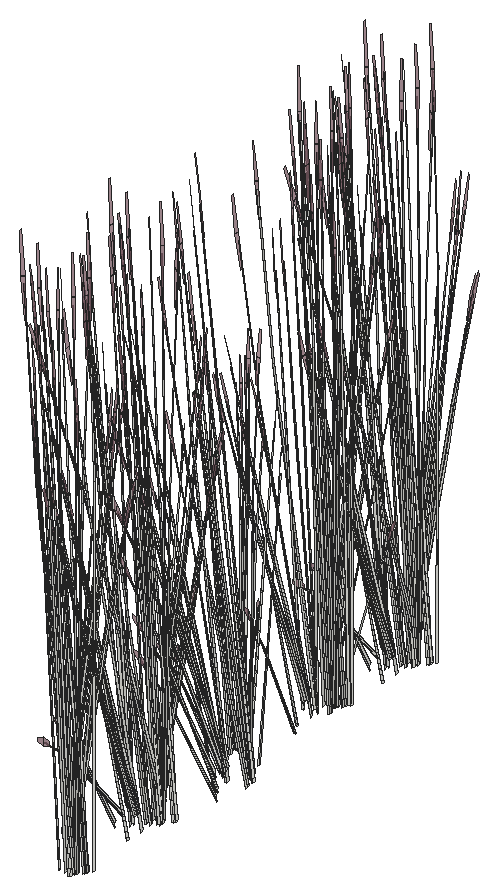
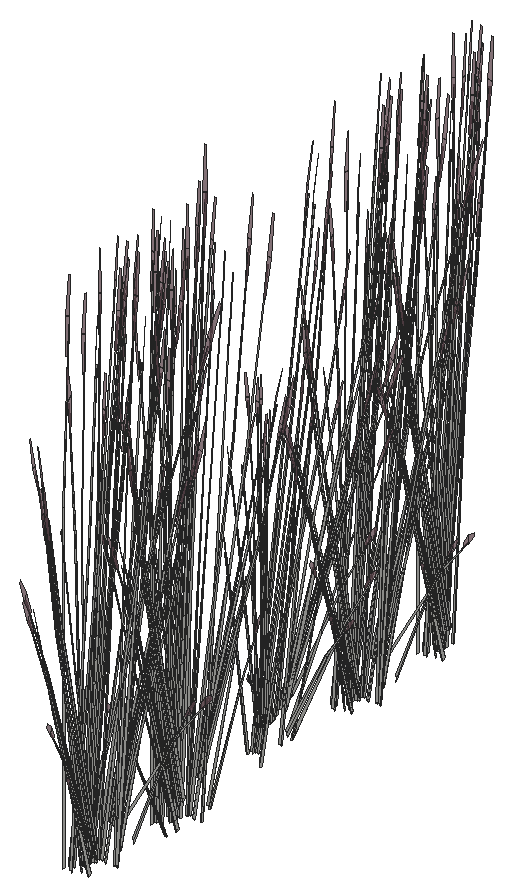
# SketchUp Ruby script. Lengths in inches.
U = 1.inch
M = Sketchup.active_model
def pt(a) = Geom::Point3d.new(a.map { |v| v * U })
def face(e, loops, mat)
  f = e.add_face(loops[0].map { |a| pt(a) })
  loops[1..].each { |l| e.add_face(l.map { |a| pt(a) }).erase! }
  f.material = f.back_material = mat if mat
  f
end
# faces: each face lists its corners as indices into pts; further lists are holes
def faces(e, pts, list, mat = nil) = list.each { |f| face(e, (f[0].is_a?(Array) ? f : [f]).map { |l| l.map { |i| pts[i] } }, mat) }
# xy, xz, yz: faces in a plane at the given z, y or x. An outline is a flat list of corners, or four numbers for a rectangle; further outlines are holes
def ring(l) = l.size == 4 ? [[l[0], l[1]], [l[2], l[1]], [l[2], l[3]], [l[0], l[3]]] : l.each_slice(2).to_a
def flat(e, list, mat, &to3) = list.each { |f| face(e, (f[0].is_a?(Array) ? f : [f]).map { |l| ring(l).map { |u, v| to3.(u, v) } }, mat) }
def xy(e, z, list, mat = nil) = flat(e, list, mat) { |x, y| [x, y, z] }
def xz(e, y, list, mat = nil) = flat(e, list, mat) { |x, z| [x, y, z] }
def yz(e, x, list, mat = nil) = flat(e, list, mat) { |y, z| [x, y, z] }
def lines(e, pts, list) = list.each { |a, b| e.add_line(pt(pts[a]), pt(pts[b])) }
# prism: a flat outline (further loops are holes) pulled along v
def prism(e, loops, v, mat = nil)
  f = face(e, loops, mat); d = Geom::Vector3d.new(v.map { |x| x * U })
  f.pushpull(f.normal.samedirection?(d) ? d.length : -d.length)
end
def box(e, o, s, mat = nil) = prism(e, [[o, [o[0] + s[0], o[1], o[2]], [o[0] + s[0], o[1] + s[1], o[2]], [o[0], o[1] + s[1], o[2]]]], [0, 0, s[2]], mat)
def at(x, y, z, deg = 0) = Geom::Transformation.translation(pt([x, y, z])) * Geom::Transformation.rotation(ORIGIN, Z_AXIS, deg.degrees)
def axes(o, x, y, z) = Geom::Transformation.new([*x, 0, *y, 0, *z, 0, *pt(o).to_a, 1])
def part(name) = M.definitions.add(name)
# library, detail: a bought-in or finely detailed component or shape, given as its bounding box
def library(name, o, s) = part(name).tap { |d| box(d.entities, o, s) }
def detail(e, o, s) = box(e.add_group.entities, o, s)
def put(e, d, t, mat = nil) = e.add_instance(d, t).tap { |i| i.material = mat if mat }
def group(e, t, mat = nil) = e.add_group.tap { |g| g.transformation = t; g.material = mat if mat }.entities
root = M.entities
M.materials.add("LightPink_Translucent").color = [144, 107, 117]
M.materials["LightPink_Translucent"].alpha = 0.75
c1 = part("blade")
p = [[2.15,0.21,22],[0,0.17,0],[0.09,0.45,0],[2.18,0.31,22],[2.29,0.31,22],[0.38,0.45,0],
  [2.48,0.24,33],[2.49,0.24,33],[2.48,0.22,33]]
faces(c1.entities,p,[[0,1,2,3],[4,5,2,3],[6,3,4,7],[8,0,3,6]])
c2 = part("seeds")
p = [[0.3,-0.1,1.38],[-0.01,-0.03,1.59],[-0.01,-0.03,0.03],[0.14,-0.07,-0.07],[0.29,-0.03,3],[0.15,0.01,3.11]]
faces(c2.entities,p,[[0,1,2,3],[1,0,4,5]],"LightPink_Translucent")
c3 = part("blade with seeds")
put(c3.entities,c1,at(0,0,0))
put(c3.entities,c2,axes([2.4,0.25,30.99],[1.5799,-0.05474,1.17369],[-0.12525,1.92788,0.29478],[-0.07173,-0.02425,1.56792]))
put(root,c3,axes([402.67,375.75,-9.47],[-0.24813,0.48978,0.41661],[-0.51557,-0.23571,-0.2005],[0,-0.1129,1.33761]))
put(root,c3,axes([402.84,375.87,-9.8],[0.64638,0.11452,0.42607],[-0.13155,0.64678,0.16719],[-0.09446,-0.06245,1.47927]))
put(root,c3,axes([402.49,376.9,-9.7],[0.54955,-0.14427,0.16428],[0.1357,0.53689,0.32672],[-0.04901,-0.07823,1.49371]))
put(root,c3,axes([403,376.33,-9.5625],[-0.09866,0.48509,0.13483],[-0.48202,-0.0842,-0.38503],[-0.08772,-0.04981,1.18024]))
put(root,c3,axes([404.125,376.93,-9.7],[0.14774,-0.54019,0.16428],[0.54062,0.15287,0.32672],[-0.09339,0.00263,1.49371]))
put(root,c3,axes([403.2,376.99,-9.95],[-0.51557,-0.24403,0],[0.24813,-0.50705,0],[0,0,1.51513]))
put(root,c3,axes([403.625,376.34,-9.7],[-0.49938,-0.43748,-0.23459],[0.42021,-0.49126,0.51337],[-0.13447,0.05118,1.56642]))
put(root,c3,axes([402.31,377.18,-9.69],[0.47863,0.27177,0.46235],[-0.28609,0.48733,0],[-0.10901,-0.0619,1.46668]))
put(root,c3,axes([403.37,376.24,-9.94],[-0.55535,0.03355,-0.41661],[-0.05022,-0.55698,0.2005],[-0.09942,0.05645,1.33761]))
put(root,c3,axes([403.99,377.54,-9.96],[-0.31576,-0.54657,-0.04789],[0.53494,-0.30375,0.48057],[-0.13182,0.05204,1.52373]))
put(root,c3,axes([403.875,376.21,-9.5625],[0.37783,0.32657,0.13483],[-0.31516,0.36844,-0.38503],[-0.08772,0.04981,1.18024]))
put(root,c3,axes([403.84,377.47,-10.11],[-0.47712,-0.13449,-0.28847],[0.12013,-0.47362,0.28847],[-0.09619,0.05462,1.29413]))
put(root,c3,axes([403.76,376.09,-9.52],[0.05959,0.62022,-0.27094],[-0.62068,0.0375,-0.46562],[-0.1093,0.08261,1.4872]))
put(root,c3,axes([403.95,377.68,-10.12],[-0.47863,0.27177,-0.46235],[-0.28609,-0.48733,0],[-0.10901,0.0619,1.46668]))
put(root,c3,axes([403.22,382.96,-7.61],[-0.07822,-0.07621,1.62908],[-0.52201,0.04832,-0.25764],[-0.08331,-0.18228,0.13065]))
put(root,c3,axes([401.8,377.02,-7.3],[0.34603,-0.28618,0.32977],[0.32756,0.32677,-0.42575],[-0.04984,0.16603,0.81462]))
put(root,c3,axes([403.77,384.25,-7.36],[-0.24409,-0.44196,-0.66157],[0.50245,-0.2463,0.07984],[-0.05708,-0.21354,0.93586]))
put(root,c3,axes([404.39,377.6,-9.79],[0.31974,0.54466,0],[-0.53494,0.30375,-0.48057],[-0.12184,0.06918,1.52448]))
put(root,c3,axes([404.12,375.44,-9.35],[-0.01397,-0.51177,1.31553],[0.63227,0.13266,0.557],[-0.14954,0.28003,1.24175]))
put(root,c3,axes([403.58,384.16,-7.64],[-0.50273,-0.13626,-0.47583],[0.17232,-0.46717,-0.36857],[-0.0461,-0.18809,0.91046]))
put(root,c3,axes([402.63,377.87,-7.6],[-0.37684,0.18473,0.05988],[-0.18445,-0.33686,0.47138],[0.03639,0.14849,0.71878]))
put(root,c3,axes([401.58,377.1,-6.97],[0.56206,0.02693,-0.12569],[-0.01536,0.50991,-0.69765],[-0.03904,0.19638,1.06006]))
put(root,c3,axes([402.58,383.87,-7.26],[0.56969,-0.13971,0.50064],[0.09887,0.54803,0.4128],[-0.13398,-0.16152,1.03595]))
put(root,c3,axes([402.76,377.83,-7.28],[-0.50393,-0.1421,0.49617],[0.17232,-0.46717,0.40911],[0.03028,0.18372,1.0267]))
put(root,c3,axes([401.84,378.54,-9.42],[-0.01324,-0.32319,1.06958],[0.33072,0.23052,0.78586],[-0.06504,0.15405,0.23558]))
put(root,c3,axes([404.01,384.14,-7.3125],[-0.50045,0.25306,-0.11324],[-0.24593,-0.44915,-0.62851],[-0.06603,-0.18927,0.95501]))
put(root,c3,axes([402.02,383.37,-9.42],[0.26677,0.18918,1.06958],[-0.38851,0.11372,0.78586],[-0.08313,-0.14539,0.23558]))
put(root,c3,axes([401.96,377.29,-7.34],[0.3661,0.36521,-0.52818],[-0.38674,0.31985,-0.40911],[-0.0557,0.18556,1.01061]))
put(root,c3,axes([401.5625,377.84,-9.37],[0.46459,-0.09625,0.0606],[0.10681,0.38778,-0.80367],[-0.02945,0.1963,0.72038]))
put(root,c3,axes([402.71,383.99,-7.6],[0.23243,-0.34529,0.05988],[0.331,0.20103,0.47138],[-0.10701,-0.1107,0.71878]))
put(root,c3,axes([402.64,385.91,-10.05],[-0.21003,-0.55738,-0.65031],[0.60499,-0.20074,-0.17068],[-0.02321,-0.18874,1.43544]))
put(root,c3,axes([401.85,377.12,-7.03],[-0.01331,0.50278,-0.73435],[-0.56035,-0.03377,0.08862],[-0.05914,0.213,1.03881]))
put(root,c3,axes([402.38,376.76,-8.39],[-0.01252,-0.20862,1.59586],[0.54251,0.1384,0.12904],[-0.03356,0.2973,0.68222]))
put(root,c3,axes([403.26,383.65,-10.02],[-0.35341,0.31182,-0.03625],[-0.32382,-0.34152,-0.16435],[-0.0228,-0.09677,0.54209]))
put(root,c3,axes([403.71,387.35,-8.9],[0.44194,0.21918,1.40854],[-0.43295,0.47219,0.557],[-0.19393,-0.27986,1.18082]))
put(root,c3,axes([402.78,384.39,-7.3],[0.07899,0.43781,0.32977],[-0.45153,0.11561,-0.42575],[-0.12128,-0.12546,0.81462]))
put(root,c3,axes([401.4,385.83,-10.12],[0,-0.54355,-0.46235],[0.57217,0,0],[0,-0.1238,1.46668]))
put(root,c3,axes([401.66,377.83,-8.87],[0.01124,-0.2806,1.43727],[0.50537,0.14821,0.19862],[-0.04379,0.29905,0.67868]))
put(root,c3,axes([401.65,385.84,-10.11],[0.35699,-0.33913,-0.28847],[0.35699,0.33913,0.28847],[0,-0.10923,1.29413]))
put(root,c3,axes([402.9,386.46,-9.52],[-0.57594,-0.25935,-0.27094],[0.27732,-0.5474,-0.46562],[-0.0181,-0.1344,1.4872]))
put(root,c3,axes([401.75,386.08,-9.83],[-0.47569,0.45698,0.2864],[-0.47598,-0.45217,-0.33981],[-0.01661,-0.12977,1.53541]))
put(root,c3,axes([403.04,387.04,-9.73],[0.13555,-0.64407,-0.21817],[0.64269,0.11227,0.47743],[-0.1123,-0.08895,1.45677]))
put(root,c3,axes([401.65,386.34,-9.69],[0,0.54355,0.46235],[-0.57217,0,0],[0,-0.1238,1.46668]))
put(root,c3,axes([403,386.78,-9.94],[-0.30722,-0.45622,-0.41661],[0.46535,-0.32126,0.2005],[-0.09942,-0.05645,1.33761]))
put(root,c3,axes([402.95,386.61,-9.47],[-0.24813,0.48978,0.41661],[-0.51557,-0.23571,-0.2005],[0,-0.1129,1.33761]))
put(root,c3,axes([403.12,386.73,-9.8],[0.64638,0.11452,0.42607],[-0.13155,0.64678,0.16719],[-0.09446,-0.06245,1.47927]))
put(root,c3,axes([402.77,387.76,-9.7],[0.54955,-0.14427,0.16428],[0.1357,0.53689,0.32672],[-0.04901,-0.07823,1.49371]))
put(root,c3,axes([403.28,387.1875,-9.5625],[-0.09866,0.48509,0.13483],[-0.48202,-0.0842,-0.38503],[-0.08772,-0.04981,1.18024]))
put(root,c3,axes([403.9,387.2,-9.7],[-0.49938,-0.43748,-0.23459],[0.42021,-0.49126,0.51337],[-0.13447,0.05118,1.56642]))
put(root,c3,axes([402.59,388.03,-9.69],[0.47863,0.27177,0.46235],[-0.28609,0.48733,0],[-0.10901,-0.0619,1.46668]))
put(root,c3,axes([403.65,387.1,-9.94],[-0.55535,0.03355,-0.41661],[-0.05022,-0.55698,0.2005],[-0.09942,0.05645,1.33761]))
put(root,c3,axes([404.27,388.4,-9.96],[-0.31576,-0.54657,-0.04789],[0.53494,-0.30375,0.48057],[-0.13182,0.05204,1.52373]))
put(root,c3,axes([404.12,388.33,-10.11],[-0.47712,-0.13449,-0.28847],[0.12013,-0.47362,0.28847],[-0.09619,0.05462,1.29413]))
put(root,c3,axes([404.63,393.81,-8.39],[0.1169,0.17452,1.59586],[-0.54019,0.14692,0.12904],[-0.12209,-0.27397,0.68222]))
put(root,c3,axes([404.04,386.95,-9.52],[0.05959,0.62022,-0.27094],[-0.62068,0.0375,-0.46562],[-0.1093,0.08261,1.4872]))
put(root,c3,axes([404.49,393.34,-9.59],[-0.03097,0.17781,1.33163],[-0.45273,0.14885,-0.28638],[-0.10583,-0.22982,0.56934]))
put(root,c3,axes([403.67,387.43,-10.08],[-0.34446,0.40855,-0.58063],[-0.42791,-0.37046,-0.15239],[-0.13803,0.10191,1.28164]))
put(root,c3,axes([404.24,388.54,-10.12],[-0.47863,0.27177,-0.46235],[-0.28609,-0.48733,0],[-0.10901,0.0619,1.46668]))
put(root,c3,axes([404.99,392.4,-7.62],[-0.00954,0.06515,1.65179],[-0.47055,0.23645,-0.15608],[-0.13847,-0.12087,0.29231]))
put(root,c3,axes([402.08,387.88,-7.3],[0.34603,-0.28618,0.32977],[0.32756,0.32677,-0.42575],[-0.04984,0.16603,0.81462]))
put(root,c3,axes([404.4,386.3,-9.35],[-0.01397,-0.51177,1.31553],[0.63227,0.13266,0.557],[-0.14954,0.28003,1.24175]))
put(root,c3,axes([404.97,394.0625,-7.36],[-0.43608,-0.26272,-0.66157],[0.30991,-0.46038,0.07984],[-0.158,-0.15687,0.93586]))
put(root,c3,axes([404.82,393.71,-7.78],[-0.07899,-0.43781,-0.32977],[0.45153,-0.11561,0.42575],[-0.12128,-0.12546,0.81462]))
put(root,c3,axes([404.12,393.63,-10.61],[-0.04954,0.0716,1.6421],[-0.50062,0.15438,-0.25086],[-0.12094,-0.14044,0.2797]))
put(root,c3,axes([404.77,394.07,-7.64],[-0.50465,0.12921,-0.47583],[-0.08828,-0.48932,-0.36857],[-0.13555,-0.14022,0.91046]))
put(root,c3,axes([401.86,387.96,-6.97],[0.56206,0.02693,-0.12569],[-0.01536,0.50991,-0.69765],[-0.03904,0.19638,1.06006]))
put(root,c3,axes([405.12,393.64,-6.94],[-0.34131,0.52108,-0.12682],[-0.49429,-0.3002,-0.70393],[-0.17182,-0.14722,1.06961]))
put(root,c3,axes([402.12,389.39,-9.42],[-0.01324,-0.32319,1.06958],[0.33072,0.23052,0.78586],[-0.06504,0.15405,0.23558]))
put(root,c3,axes([402.24,388.15,-7.34],[0.3661,0.36521,-0.52818],[-0.38674,0.31985,-0.40911],[-0.0557,0.18556,1.01061]))
put(root,c3,axes([401.84,388.7,-9.37],[0.46459,-0.09625,0.0606],[0.10681,0.38778,-0.80367],[-0.02945,0.1963,0.72038]))
put(root,c3,axes([403.73,394.36,-7.26],[0.42234,-0.40113,0.50064],[0.36424,0.42599,0.4128],[-0.19815,-0.07399,1.03595]))
put(root,c3,axes([402.13,387.98,-7.03],[-0.01331,0.50278,-0.73435],[-0.56035,-0.03377,0.08862],[-0.05914,0.213,1.03881]))
put(root,c3,axes([400.66,389.3,-7.62],[0.05802,-0.03282,1.65179],[0.47954,0.21828,-0.15608],[-0.01127,0.18175,0.29231]))
put(root,c3,axes([402.66,387.625,-8.39],[-0.01252,-0.20862,1.59586],[0.54251,0.1384,0.12904],[-0.03356,0.2973,0.68222]))
put(root,c3,axes([403.93,394.35,-7.6],[0.02575,-0.41332,0.05988],[0.38885,0.01133,0.47138],[-0.14895,-0.04325,0.71878]))
put(root,c3,axes([403.81,393.9,-10.02],[-0.14753,0.44383,-0.03625],[-0.45406,-0.13653,-0.16435],[-0.06894,-0.07259,0.54209]))
put(root,c3,axes([403.5625,395.93,-9.79],[-0.63949,0,0],[0,-0.60749,-0.48057],[0,-0.13836,1.52448]))
put(root,c3,axes([401.94,388.6875,-8.87],[0.01124,-0.2806,1.43727],[0.50537,0.14821,0.19862],[-0.04379,0.29905,0.67868]))
put(root,c3,axes([404.19,394.66,-7.3],[0.29098,0.34031,0.32977],[-0.33226,0.32215,-0.42575],[-0.16881,-0.04902,0.81462]))
put(root,c3,axes([403.08,395.3,-9.42],[0.3265,-0.03889,1.06958],[-0.20711,0.3427,0.78586],[-0.16135,-0.05141,0.23558]))
put(root,c3,axes([405.03,396.64,-10.08],[-0.53199,-0.08911,-0.58063],[0.11226,-0.54969,-0.15239],[-0.15876,-0.06661,1.28164]))
put(root,c3,axes([404.46,397.47,-10.11],[-0.12013,-0.47362,-0.28847],[0.47712,-0.13449,0.28847],[-0.09619,-0.05462,1.29413]))
put(root,c3,axes([404.33,397.68,-10.12],[-0.47863,-0.27177,-0.46235],[0.28609,-0.48733,0],[-0.10901,-0.0619,1.46668]))
put(root,c3,axes([405.63,396.72,-9.52],[-0.51635,0.36087,-0.27094],[-0.34336,-0.5099,-0.46562],[-0.1274,-0.05178,1.4872]))
put(root,c3,axes([403.71,395.62,-7.3],[0.42502,0.15163,0.32977],[-0.12396,0.44238,-0.42575],[-0.17112,0.04056,0.81462]))
put(root,c3,axes([404.62,398,-9.79],[-0.31974,0.54466,0],[-0.53494,-0.30375,-0.48057],[-0.12184,-0.06918,1.52448]))
put(root,c3,axes([403.48,396.84,-7.59],[-0.12683,-0.50025,0.447],[0.49754,-0.08682,0.36857],[-0.14663,0.11765,0.92496]))
put(root,c3,axes([403.38,396.75,-7.6],[-0.35109,-0.22859,0.05988],[0.2044,-0.32553,0.47138],[-0.11256,0.10524,0.71878]))
put(root,c3,axes([403.78,396.68,-7.3],[0.44516,-0.07768,0.32977],[0.11755,0.44407,-0.42575],[-0.12757,0.11927,0.81462]))
put(root,c3,axes([402.77,397.9375,-6.74],[0.45129,0.14509,-0.06041],[-0.13882,0.44656,-0.27392],[-0.07381,0.0678,0.90349]))
put(root,c3,axes([403.55,396.64,-7.3125],[0.47307,0.29971,-0.11324],[-0.27254,0.43404,-0.62851],[-0.13365,0.15087,0.95501]))
put(root,c3,axes([403.79,396.99,-7.64],[0.13138,0.49631,-0.47583],[-0.49754,0.08682,-0.36857],[-0.14258,0.13331,0.91046]))
put(root,c3,axes([404.07,397.82,-7.6],[-0.42027,-0.02533,0.05988],[0.01152,-0.38243,0.47138],[-0.04398,0.14649,0.71878]))
put(root,c3,axes([403.18,398.26,-10.61],[0.0686,0.0543,1.6421],[0.11632,0.50315,-0.25086],[-0.15204,0.10729,0.2797]))
put(root,c3,axes([404.2,397.86,-7.59],[-0.36417,-0.37086,0.447],[0.38674,-0.31985,0.36857],[-0.06718,0.174,0.92496]))
put(root,c3,axes([404.09,396.91,-8.39],[0.09522,-0.18683,1.59586],[0.39947,0.38663,0.12904],[-0.18021,0.24097,0.68222]))
put(root,c3,axes([404.2,397.97,-7.78],[-0.34603,0.28618,-0.32977],[-0.32756,-0.32677,0.42575],[-0.04984,0.16603,0.81462]))
put(root,c3,axes([403.01,397.88,-7.61],[-0.01271,0.10756,1.62908],[0.36076,0.37419,-0.25764],[-0.09444,0.17695,0.13065]))
put(root,c3,axes([402.68,407.0625,-7.36],[-0.24409,-0.44196,-0.66157],[0.50245,-0.2463,0.07984],[-0.05708,-0.21354,0.93586]))
put(root,c3,axes([402.26,406.08,-10.61],[-0.08578,0.01958,1.6421],[-0.47437,-0.22044,-0.25086],[0.00796,-0.18387,0.2797]))
put(root,c3,axes([404.04,398.79,-9.59],[0.16138,-0.08575,1.33163],[0.39845,0.25854,-0.28638],[-0.1186,0.22371,0.56934]))
put(root,c3,axes([402.73,406.6875,-7.78],[0.15418,-0.41799,-0.32977],[0.44981,0.12192,0.42575],[-0.04124,-0.16829,0.81462]))
put(root,c3,axes([402.5,406.97,-7.64],[-0.50273,-0.13626,-0.47583],[0.17232,-0.46717,-0.36857],[-0.0461,-0.18809,0.91046]))
put(root,c3,axes([402.93,406.95,-7.3125],[-0.50045,0.25306,-0.11324],[-0.24593,-0.44915,-0.62851],[-0.06603,-0.18927,0.95501]))
put(root,c3,axes([401.55,408.72,-10.05],[-0.21003,-0.55738,-0.65031],[0.60499,-0.20074,-0.17068],[-0.02321,-0.18874,1.43544]))
put(root,c3,axes([402.78,407.13,-7.3],[-0.15418,0.41799,0.32977],[-0.44981,-0.12192,-0.42575],[-0.04124,-0.16829,0.81462]))
put(root,c3,axes([402.17,406.47,-10.02],[-0.35341,0.31182,-0.03625],[-0.32382,-0.34152,-0.16435],[-0.0228,-0.09677,0.54209]))
put(root,c3,axes([401.875,408.87,-9.94],[0.24813,-0.48978,-0.41661],[0.51557,0.23571,0.2005],[0,-0.1129,1.33761]))
put(root,c3,axes([400.5625,408.66,-10.11],[0.35699,-0.33913,-0.28847],[0.35699,0.33913,0.28847],[0,-0.10923,1.29413]))
put(root,c3,axes([401.8125,409.27,-9.52],[-0.57594,-0.25935,-0.27094],[0.27732,-0.5474,-0.46562],[-0.0181,-0.1344,1.4872]))
put(root,c3,axes([401.98,408.95,-9.8],[0.22235,0.6078,0.42607],[-0.63531,0.21135,0.16719],[0.00776,-0.11168,1.47927]))
put(root,c3,axes([401.86,409.42,-9.47],[-0.24813,0.48978,0.41661],[-0.51557,-0.23571,-0.2005],[0,-0.1129,1.33761]))
put(root,c3,axes([402.9375,409.48,-9.86],[-0.47569,-0.46784,-0.05709],[0.47598,-0.46812,0],[-0.01661,-0.01634,1.63492]))
put(root,c3,axes([402.03,409.54,-9.8],[0.64638,0.11452,0.42607],[-0.13155,0.64678,0.16719],[-0.09446,-0.06245,1.47927]))
put(root,c3,axes([401.68,410.57,-9.7],[0.54955,-0.14427,0.16428],[0.1357,0.53689,0.32672],[-0.04901,-0.07823,1.49371]))
put(root,c3,axes([402.51,410.45,-9.95],[-0.16686,-0.46861,0],[0.47648,-0.16411,0],[0,0,1.4375]))
put(root,c3,axes([403.32,410.6,-9.7],[0.14774,-0.54019,0.16428],[0.54062,0.15287,0.32672],[-0.09339,0.00263,1.49371]))
put(root,c3,axes([402.39,410.66,-9.95],[-0.51557,-0.24403,0],[0.24813,-0.50705,0],[0,0,1.51513]))
put(root,c3,axes([403.0625,409.65,-9.47],[0.55535,-0.03355,0.41661],[0.05022,0.55698,-0.2005],[-0.09942,0.05645,1.33761]))
put(root,c3,axes([403.07,409.89,-9.5625],[0.37783,0.32657,0.13483],[-0.31516,0.36844,-0.38503],[-0.08772,0.04981,1.18024]))
put(root,c3,axes([403.47,410.89,-9.69],[0.47863,-0.27177,0.46235],[0.28609,0.48733,0],[-0.10901,0.0619,1.46668]))
put(root,c3,axes([403.04,411.14,-10.11],[-0.47712,-0.13449,-0.28847],[0.12013,-0.47362,0.28847],[-0.09619,0.05462,1.29413]))
put(root,c3,axes([403.09,415.38,-7.61],[-0.07822,-0.07621,1.62908],[-0.52201,0.04832,-0.25764],[-0.08331,-0.18228,0.13065]))
put(root,c3,axes([403.63,416.67,-7.36],[-0.24409,-0.44196,-0.66157],[0.50245,-0.2463,0.07984],[-0.05708,-0.21354,0.93586]))
put(root,c3,axes([402.96,409.77,-9.52],[0.05959,0.62022,-0.27094],[-0.62068,0.0375,-0.46562],[-0.1093,0.08261,1.4872]))
put(root,c3,axes([403.18,409.52,-9.94],[-0.24813,0.48978,-0.41661],[-0.51557,-0.23571,0.2005],[0,0.1129,1.33761]))
put(root,c3,axes([403.2,410.93,-9.83],[0.64025,0.17667,0.2864],[-0.16018,0.63149,-0.33981],[-0.10597,0.07904,1.53541]))
put(root,c3,axes([403.45,416.58,-7.64],[-0.50273,-0.13626,-0.47583],[0.17232,-0.46717,-0.36857],[-0.0461,-0.18809,0.91046]))
put(root,c3,axes([402.45,416.28,-7.26],[0.56969,-0.13971,0.50064],[0.09887,0.54803,0.4128],[-0.13398,-0.16152,1.03595]))
put(root,c3,axes([400.99,410.69,-7.3],[0.34603,-0.28618,0.32977],[0.32756,0.32677,-0.42575],[-0.04984,0.16603,0.81462]))
put(root,c3,axes([403.58,411.27,-9.79],[0.31974,0.54466,0],[-0.53494,0.30375,-0.48057],[-0.12184,0.06918,1.52448]))
put(root,c3,axes([403.88,416.55,-7.3125],[-0.50045,0.25306,-0.11324],[-0.24593,-0.44915,-0.62851],[-0.06603,-0.18927,0.95501]))
put(root,c3,axes([401.89,415.79,-9.42],[0.26677,0.18918,1.06958],[-0.38851,0.11372,0.78586],[-0.08313,-0.14539,0.23558]))
put(root,c3,axes([403.3125,409.11,-9.35],[-0.01397,-0.51177,1.31553],[0.63227,0.13266,0.557],[-0.14954,0.28003,1.24175]))
put(root,c3,axes([402.58,416.4,-7.6],[0.23243,-0.34529,0.05988],[0.331,0.20103,0.47138],[-0.10701,-0.1107,0.71878]))
put(root,c3,axes([402.51,418.33,-10.05],[-0.21003,-0.55738,-0.65031],[0.60499,-0.20074,-0.17068],[-0.02321,-0.18874,1.43544]))
put(root,c3,axes([403.73,416.73,-7.3],[-0.15418,0.41799,0.32977],[-0.44981,-0.12192,-0.42575],[-0.04124,-0.16829,0.81462]))
put(root,c3,axes([401.82,411.54,-7.6],[-0.37684,0.18473,0.05988],[-0.18445,-0.33686,0.47138],[0.03639,0.14849,0.71878]))
put(root,c3,axes([400.77,410.77,-6.97],[0.56206,0.02693,-0.12569],[-0.01536,0.50991,-0.69765],[-0.03904,0.19638,1.06006]))
put(root,c3,axes([401.96,411.5,-7.28],[-0.50393,-0.1421,0.49617],[0.17232,-0.46717,0.40911],[0.03028,0.18372,1.0267]))
put(root,c3,axes([403.125,416.07,-10.02],[-0.35341,0.31182,-0.03625],[-0.32382,-0.34152,-0.16435],[-0.0228,-0.09677,0.54209]))
put(root,c3,axes([401.9,411.4375,-10.61],[0.08277,-0.02958,1.6421],[0.49786,0.16279,-0.25086],[0.01456,0.18348,0.2797]))
put(root,c3,axes([401.16,410.96,-7.34],[0.3661,0.36521,-0.52818],[-0.38674,0.31985,-0.40911],[-0.0557,0.18556,1.01061]))
put(root,c3,axes([400.76,411.51,-9.37],[0.46459,-0.09625,0.0606],[0.10681,0.38778,-0.80367],[-0.02945,0.1963,0.72038]))
put(root,c3,axes([403.58,419.76,-8.9],[0.44194,0.21918,1.40854],[-0.43295,0.47219,0.557],[-0.19393,-0.27986,1.18082]))
put(root,c3,axes([402.65,416.8,-7.3],[0.07899,0.43781,0.32977],[-0.45153,0.11561,-0.42575],[-0.12128,-0.12546,0.81462]))
put(root,c3,axes([401.27,418.25,-10.12],[0,-0.54355,-0.46235],[0.57217,0,0],[0,-0.1238,1.46668]))
put(root,c3,axes([402.01,411.6,-7.78],[-0.15418,0.41799,-0.32977],[-0.44981,-0.12192,0.42575],[0.04124,0.16829,0.81462]))
put(root,c3,axes([401.57,410.4375,-8.39],[-0.01252,-0.20862,1.59586],[0.54251,0.1384,0.12904],[-0.03356,0.2973,0.68222]))
put(root,c3,axes([401.51,418.26,-10.11],[0.35699,-0.33913,-0.28847],[0.35699,0.33913,0.28847],[0,-0.10923,1.29413]))
put(root,c3,axes([402.76,418.875,-9.52],[-0.57594,-0.25935,-0.27094],[0.27732,-0.5474,-0.46562],[-0.0181,-0.1344,1.4872]))
put(root,c3,axes([401.62,418.5,-9.83],[-0.47569,0.45698,0.2864],[-0.47598,-0.45217,-0.33981],[-0.01661,-0.12977,1.53541]))
put(root,c3,axes([402.91,419.45,-9.73],[0.13555,-0.64407,-0.21817],[0.64269,0.11227,0.47743],[-0.1123,-0.08895,1.45677]))
put(root,c3,axes([401.51,418.75,-9.69],[0,0.54355,0.46235],[-0.57217,0,0],[0,-0.1238,1.46668]))
put(root,c3,axes([402.86,419.19,-9.94],[-0.30722,-0.45622,-0.41661],[0.46535,-0.32126,0.2005],[-0.09942,-0.05645,1.33761]))
put(root,c3,axes([402.82,419.03,-9.47],[-0.24813,0.48978,0.41661],[-0.51557,-0.23571,-0.2005],[0,-0.1129,1.33761]))
put(root,c3,axes([402.98,419.14,-9.8],[0.64638,0.11452,0.42607],[-0.13155,0.64678,0.16719],[-0.09446,-0.06245,1.47927]))
put(root,c3,axes([402.64,420.18,-9.7],[0.54955,-0.14427,0.16428],[0.1357,0.53689,0.32672],[-0.04901,-0.07823,1.49371]))
put(root,c3,axes([403.14,419.6,-9.5625],[-0.09866,0.48509,0.13483],[-0.48202,-0.0842,-0.38503],[-0.08772,-0.04981,1.18024]))
put(root,c3,axes([403.34,420.26,-9.95],[-0.51557,-0.24403,0],[0.24813,-0.50705,0],[0,0,1.51513]))
put(root,c3,axes([403.77,419.61,-9.7],[-0.49938,-0.43748,-0.23459],[0.42021,-0.49126,0.51337],[-0.13447,0.05118,1.56642]))
put(root,c3,axes([402.46,420.45,-9.69],[0.47863,0.27177,0.46235],[-0.28609,0.48733,0],[-0.10901,-0.0619,1.46668]))
put(root,c3,axes([403.52,419.52,-9.94],[-0.55535,0.03355,-0.41661],[-0.05022,-0.55698,0.2005],[-0.09942,0.05645,1.33761]))
put(root,c3,axes([404.13,420.81,-9.96],[-0.31576,-0.54657,-0.04789],[0.53494,-0.30375,0.48057],[-0.13182,0.05204,1.52373]))
put(root,c3,axes([403.99,420.74,-10.11],[-0.47712,-0.13449,-0.28847],[0.12013,-0.47362,0.28847],[-0.09619,0.05462,1.29413]))
put(root,c3,axes([403.91,419.37,-9.52],[0.05959,0.62022,-0.27094],[-0.62068,0.0375,-0.46562],[-0.1093,0.08261,1.4872]))
put(root,c3,axes([404.1,420.96,-10.12],[-0.47863,0.27177,-0.46235],[-0.28609,-0.48733,0],[-0.10901,0.0619,1.46668]))
put(root,c3,axes([401.94,420.29,-7.3],[0.34603,-0.28618,0.32977],[0.32756,0.32677,-0.42575],[-0.04984,0.16603,0.81462]))
put(root,c3,axes([404.54,420.87,-9.79],[0.31974,0.54466,0],[-0.53494,0.30375,-0.48057],[-0.12184,0.06918,1.52448]))
put(root,c3,axes([404.26,418.72,-9.35],[-0.01397,-0.51177,1.31553],[0.63227,0.13266,0.557],[-0.14954,0.28003,1.24175]))
put(root,c3,axes([401.72,420.37,-6.97],[0.56206,0.02693,-0.12569],[-0.01536,0.50991,-0.69765],[-0.03904,0.19638,1.06006]))
put(root,c3,axes([402.91,421.11,-7.28],[-0.50393,-0.1421,0.49617],[0.17232,-0.46717,0.40911],[0.03028,0.18372,1.0267]))
put(root,c3,axes([401.98,421.81,-9.42],[-0.01324,-0.32319,1.06958],[0.33072,0.23052,0.78586],[-0.06504,0.15405,0.23558]))
put(root,c3,axes([402.11,420.5625,-7.34],[0.3661,0.36521,-0.52818],[-0.38674,0.31985,-0.40911],[-0.0557,0.18556,1.01061]))
put(root,c3,axes([401.71,421.11,-9.37],[0.46459,-0.09625,0.0606],[0.10681,0.38778,-0.80367],[-0.02945,0.1963,0.72038]))
put(root,c3,axes([401.99,420.4,-7.03],[-0.01331,0.50278,-0.73435],[-0.56035,-0.03377,0.08862],[-0.05914,0.213,1.03881]))
put(root,c3,axes([400.53,421.72,-7.62],[0.05802,-0.03282,1.65179],[0.47954,0.21828,-0.15608],[-0.01127,0.18175,0.29231]))
put(root,c3,axes([402.52,420.04,-8.39],[-0.01252,-0.20862,1.59586],[0.54251,0.1384,0.12904],[-0.03356,0.2973,0.68222]))
put(root,c3,axes([401.81,421.1,-8.87],[0.01124,-0.2806,1.43727],[0.50537,0.14821,0.19862],[-0.04379,0.29905,0.67868]))
